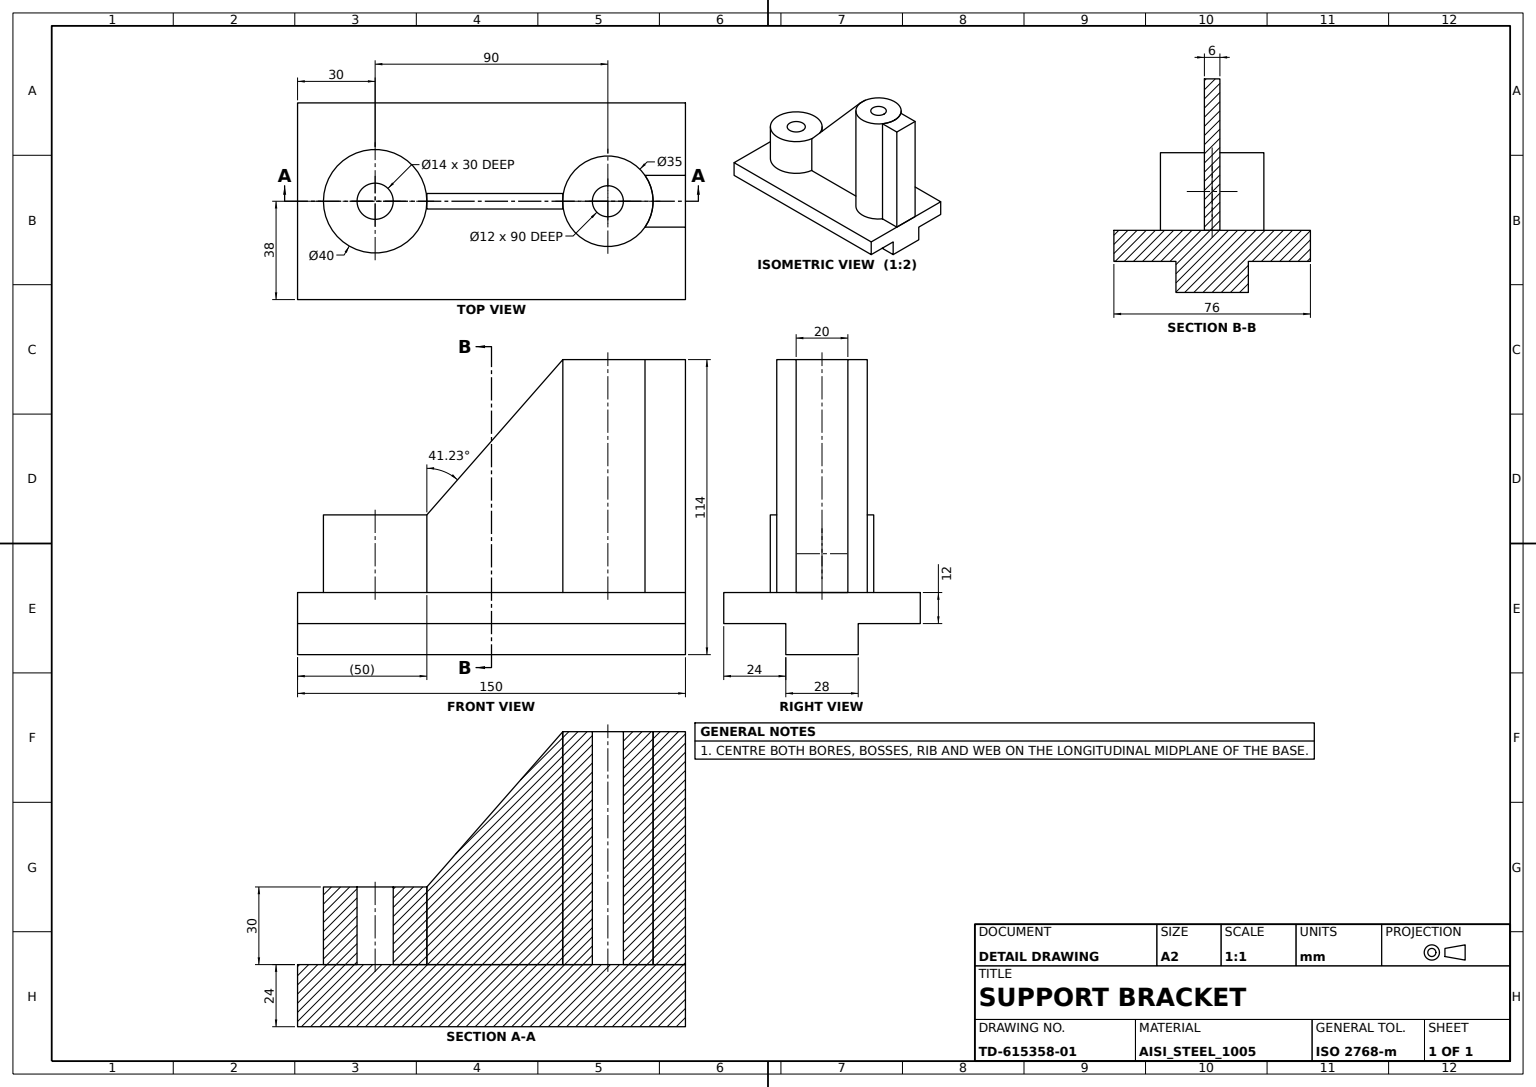
ISO-10303-21;
HEADER;
FILE_DESCRIPTION((''),'2;1');
FILE_NAME('','',(''),(''),'','','');
FILE_SCHEMA(('AUTOMOTIVE_DESIGN'));
ENDSEC;
DATA;
#1=APPLICATION_CONTEXT('');
#2=PRODUCT_CONTEXT('',#1,'mechanical');
#3=PRODUCT('','','',(#2));
#4=PRODUCT_DEFINITION_FORMATION('','',#3);
#5=PRODUCT_DEFINITION_CONTEXT('',#1,'design');
#6=PRODUCT_DEFINITION('','',#4,#5);
#7=PRODUCT_DEFINITION_SHAPE('','',#6);
#8=(LENGTH_UNIT()NAMED_UNIT(*)SI_UNIT(.MILLI.,.METRE.));
#9=(NAMED_UNIT(*)PLANE_ANGLE_UNIT()SI_UNIT($,.RADIAN.));
#10=(NAMED_UNIT(*)SI_UNIT($,.STERADIAN.)SOLID_ANGLE_UNIT());
#11=UNCERTAINTY_MEASURE_WITH_UNIT(LENGTH_MEASURE(0.005),#8,'distance_accuracy_value','');
#12=(GEOMETRIC_REPRESENTATION_CONTEXT(3)GLOBAL_UNCERTAINTY_ASSIGNED_CONTEXT((#11))GLOBAL_UNIT_ASSIGNED_CONTEXT((#8,#9,#10))REPRESENTATION_CONTEXT('',''));
#13=CARTESIAN_POINT('',(10.,-15.638593,114.));
#14=VERTEX_POINT('',#13);
#15=CARTESIAN_POINT('',(-10.,-15.638593,114.));
#16=VERTEX_POINT('',#15);
#17=CARTESIAN_POINT('',(0.,-30.,114.));
#18=DIRECTION('',(0.,0.,1.));
#19=DIRECTION('',(0.,1.,0.));
#20=AXIS2_PLACEMENT_3D('',#17,#18,#19);
#21=CIRCLE('',#20,17.5);
#22=EDGE_CURVE('',#14,#16,#21,.T.);
#23=ORIENTED_EDGE('',*,*,#22,.F.);
#24=CARTESIAN_POINT('',(10.,0.,114.));
#25=VERTEX_POINT('',#24);
#26=DIRECTION('',(0.,-1.,0.));
#27=VECTOR('',#26,1000.);
#28=LINE('',#24,#27);
#29=EDGE_CURVE('',#25,#14,#28,.T.);
#30=ORIENTED_EDGE('',*,*,#29,.F.);
#31=CARTESIAN_POINT('',(-10.,0.,114.));
#32=VERTEX_POINT('',#31);
#33=DIRECTION('',(1.,0.,0.));
#34=VECTOR('',#33,1000.);
#35=LINE('',#31,#34);
#36=EDGE_CURVE('',#32,#25,#35,.T.);
#37=ORIENTED_EDGE('',*,*,#36,.F.);
#38=VECTOR('',#19,1000.);
#39=LINE('',#15,#38);
#40=EDGE_CURVE('',#16,#32,#39,.T.);
#41=ORIENTED_EDGE('',*,*,#40,.F.);
#42=EDGE_LOOP('',(#23,#30,#37,#41));
#43=FACE_BOUND('',#42,.T.);
#44=AXIS2_PLACEMENT_3D('',#17,#18,#33);
#45=PLANE('',#44);
#46=ADVANCED_FACE('',(#43),#45,.T.);
#47=CARTESIAN_POINT('',(10.,-15.638593,24.));
#48=VERTEX_POINT('',#47);
#49=VECTOR('',#18,1000.);
#50=LINE('',#47,#49);
#51=EDGE_CURVE('',#48,#14,#50,.T.);
#52=ORIENTED_EDGE('',*,*,#51,.T.);
#53=ORIENTED_EDGE('',*,*,#22,.T.);
#54=CARTESIAN_POINT('',(-10.,-15.638593,24.));
#55=VERTEX_POINT('',#54);
#56=LINE('',#54,#49);
#57=EDGE_CURVE('',#55,#16,#56,.T.);
#58=ORIENTED_EDGE('',*,*,#57,.F.);
#59=CARTESIAN_POINT('',(0.,-30.,24.));
#60=AXIS2_PLACEMENT_3D('',#59,#18,#19);
#61=CIRCLE('',#60,17.5);
#62=EDGE_CURVE('',#48,#55,#61,.T.);
#63=ORIENTED_EDGE('',*,*,#62,.F.);
#64=EDGE_LOOP('',(#52,#53,#58,#63));
#65=FACE_BOUND('',#64,.T.);
#66=AXIS2_PLACEMENT_3D('',#59,#18,#33);
#67=CYLINDRICAL_SURFACE('',#66,17.5);
#68=ADVANCED_FACE('',(#65),#67,.F.);
#69=CARTESIAN_POINT('',(10.,0.,24.));
#70=VERTEX_POINT('',#69);
#71=LINE('',#69,#49);
#72=EDGE_CURVE('',#70,#25,#71,.T.);
#73=ORIENTED_EDGE('',*,*,#72,.T.);
#74=ORIENTED_EDGE('',*,*,#29,.T.);
#75=ORIENTED_EDGE('',*,*,#51,.F.);
#76=LINE('',#69,#27);
#77=EDGE_CURVE('',#70,#48,#76,.T.);
#78=ORIENTED_EDGE('',*,*,#77,.F.);
#79=EDGE_LOOP('',(#73,#74,#75,#78));
#80=FACE_BOUND('',#79,.T.);
#81=DIRECTION('',(-1.,0.,0.));
#82=AXIS2_PLACEMENT_3D('',#69,#81,#26);
#83=PLANE('',#82);
#84=ADVANCED_FACE('',(#80),#83,.F.);
#85=ORIENTED_EDGE('',*,*,#36,.T.);
#86=ORIENTED_EDGE('',*,*,#72,.F.);
#87=CARTESIAN_POINT('',(-10.,0.,24.));
#88=VERTEX_POINT('',#87);
#89=LINE('',#87,#34);
#90=EDGE_CURVE('',#88,#70,#89,.T.);
#91=ORIENTED_EDGE('',*,*,#90,.F.);
#92=LINE('',#87,#49);
#93=EDGE_CURVE('',#88,#32,#92,.T.);
#94=ORIENTED_EDGE('',*,*,#93,.T.);
#95=EDGE_LOOP('',(#85,#86,#91,#94));
#96=FACE_BOUND('',#95,.T.);
#97=DIRECTION('',(0.,0.,-1.));
#98=AXIS2_PLACEMENT_3D('',#87,#26,#97);
#99=PLANE('',#98);
#100=ADVANCED_FACE('',(#96),#99,.F.);
#101=LINE('',#54,#38);
#102=EDGE_CURVE('',#55,#88,#101,.T.);
#103=ORIENTED_EDGE('',*,*,#102,.F.);
#104=ORIENTED_EDGE('',*,*,#57,.T.);
#105=ORIENTED_EDGE('',*,*,#40,.T.);
#106=ORIENTED_EDGE('',*,*,#93,.F.);
#107=EDGE_LOOP('',(#103,#104,#105,#106));
#108=FACE_BOUND('',#107,.T.);
#109=AXIS2_PLACEMENT_3D('',#54,#33,#19);
#110=PLANE('',#109);
#111=ADVANCED_FACE('',(#108),#110,.F.);
#112=ORIENTED_EDGE('',*,*,#102,.T.);
#113=ORIENTED_EDGE('',*,*,#90,.T.);
#114=ORIENTED_EDGE('',*,*,#77,.T.);
#115=ORIENTED_EDGE('',*,*,#62,.T.);
#116=EDGE_LOOP('',(#112,#113,#114,#115));
#117=FACE_BOUND('',#116,.T.);
#118=PLANE('',#66);
#119=ADVANCED_FACE('',(#117),#118,.F.);
#120=CLOSED_SHELL('',(#46,#68,#84,#100,#111,#119));
#121=MANIFOLD_SOLID_BREP('',#120);
#122=CARTESIAN_POINT('',(-3.,-100.,54.));
#123=VERTEX_POINT('',#122);
#124=CARTESIAN_POINT('',(-3.,-47.413188,114.));
#125=VERTEX_POINT('',#124);
#126=DIRECTION('',(0.,0.659120652,0.75203721));
#127=VECTOR('',#126,1000.);
#128=LINE('',#122,#127);
#129=EDGE_CURVE('',#123,#125,#128,.T.);
#130=ORIENTED_EDGE('',*,*,#129,.F.);
#131=CARTESIAN_POINT('',(3.,-100.,54.));
#132=VERTEX_POINT('',#131);
#133=VECTOR('',#81,1000.);
#134=LINE('',#131,#133);
#135=EDGE_CURVE('',#132,#123,#134,.T.);
#136=ORIENTED_EDGE('',*,*,#135,.F.);
#137=CARTESIAN_POINT('',(3.,-47.413188,114.));
#138=VERTEX_POINT('',#137);
#139=LINE('',#131,#127);
#140=EDGE_CURVE('',#132,#138,#139,.T.);
#141=ORIENTED_EDGE('',*,*,#140,.T.);
#142=LINE('',#137,#133);
#143=EDGE_CURVE('',#138,#125,#142,.T.);
#144=ORIENTED_EDGE('',*,*,#143,.T.);
#145=EDGE_LOOP('',(#130,#136,#141,#144));
#146=FACE_BOUND('',#145,.T.);
#147=DIRECTION('',(0.,-0.75203721,0.659120652));
#148=DIRECTION('',(0.,-0.659120652,-0.75203721));
#149=AXIS2_PLACEMENT_3D('',#131,#147,#148);
#150=PLANE('',#149);
#151=ADVANCED_FACE('',(#146),#150,.T.);
#152=CARTESIAN_POINT('',(-3.,-100.,24.));
#153=VERTEX_POINT('',#152);
#154=LINE('',#152,#49);
#155=EDGE_CURVE('',#153,#123,#154,.T.);
#156=ORIENTED_EDGE('',*,*,#155,.T.);
#157=ORIENTED_EDGE('',*,*,#129,.T.);
#158=CARTESIAN_POINT('',(-3.,-47.413188,24.));
#159=VERTEX_POINT('',#158);
#160=VECTOR('',#97,1000.);
#161=LINE('',#124,#160);
#162=EDGE_CURVE('',#125,#159,#161,.T.);
#163=ORIENTED_EDGE('',*,*,#162,.T.);
#164=LINE('',#158,#27);
#165=EDGE_CURVE('',#159,#153,#164,.T.);
#166=ORIENTED_EDGE('',*,*,#165,.T.);
#167=EDGE_LOOP('',(#156,#157,#163,#166));
#168=FACE_BOUND('',#167,.T.);
#169=CARTESIAN_POINT('',(-3.,0.,0.));
#170=AXIS2_PLACEMENT_3D('',#169,#33,#97);
#171=PLANE('',#170);
#172=ADVANCED_FACE('',(#168),#171,.F.);
#173=ORIENTED_EDGE('',*,*,#140,.F.);
#174=CARTESIAN_POINT('',(3.,-100.,24.));
#175=VERTEX_POINT('',#174);
#176=LINE('',#174,#49);
#177=EDGE_CURVE('',#175,#132,#176,.T.);
#178=ORIENTED_EDGE('',*,*,#177,.F.);
#179=CARTESIAN_POINT('',(3.,-47.413188,24.));
#180=VERTEX_POINT('',#179);
#181=LINE('',#179,#27);
#182=EDGE_CURVE('',#180,#175,#181,.T.);
#183=ORIENTED_EDGE('',*,*,#182,.F.);
#184=LINE('',#137,#160);
#185=EDGE_CURVE('',#138,#180,#184,.T.);
#186=ORIENTED_EDGE('',*,*,#185,.F.);
#187=EDGE_LOOP('',(#173,#178,#183,#186));
#188=FACE_BOUND('',#187,.T.);
#189=CARTESIAN_POINT('',(3.,0.,0.));
#190=AXIS2_PLACEMENT_3D('',#189,#33,#97);
#191=PLANE('',#190);
#192=ADVANCED_FACE('',(#188),#191,.T.);
#193=LINE('',#179,#133);
#194=EDGE_CURVE('',#180,#159,#193,.T.);
#195=ORIENTED_EDGE('',*,*,#194,.T.);
#196=ORIENTED_EDGE('',*,*,#162,.F.);
#197=ORIENTED_EDGE('',*,*,#143,.F.);
#198=ORIENTED_EDGE('',*,*,#185,.T.);
#199=EDGE_LOOP('',(#195,#196,#197,#198));
#200=FACE_BOUND('',#199,.T.);
#201=AXIS2_PLACEMENT_3D('',#137,#19,#18);
#202=PLANE('',#201);
#203=ADVANCED_FACE('',(#200),#202,.T.);
#204=ORIENTED_EDGE('',*,*,#194,.F.);
#205=ORIENTED_EDGE('',*,*,#182,.T.);
#206=LINE('',#174,#133);
#207=EDGE_CURVE('',#175,#153,#206,.T.);
#208=ORIENTED_EDGE('',*,*,#207,.T.);
#209=ORIENTED_EDGE('',*,*,#165,.F.);
#210=EDGE_LOOP('',(#204,#205,#208,#209));
#211=FACE_BOUND('',#210,.T.);
#212=AXIS2_PLACEMENT_3D('',#179,#97,#81);
#213=PLANE('',#212);
#214=ADVANCED_FACE('',(#211),#213,.T.);
#215=ORIENTED_EDGE('',*,*,#177,.T.);
#216=ORIENTED_EDGE('',*,*,#135,.T.);
#217=ORIENTED_EDGE('',*,*,#155,.F.);
#218=ORIENTED_EDGE('',*,*,#207,.F.);
#219=EDGE_LOOP('',(#215,#216,#217,#218));
#220=FACE_BOUND('',#219,.T.);
#221=AXIS2_PLACEMENT_3D('',#174,#26,#97);
#222=PLANE('',#221);
#223=ADVANCED_FACE('',(#220),#222,.T.);
#224=CLOSED_SHELL('',(#151,#172,#192,#203,#214,#223));
#225=MANIFOLD_SOLID_BREP('',#224);
#226=CARTESIAN_POINT('',(0.,-113.,24.));
#227=VERTEX_POINT('',#226);
#228=CARTESIAN_POINT('',(0.,-120.,24.));
#229=AXIS2_PLACEMENT_3D('',#228,#18,#19);
#230=CIRCLE('',#229,7.);
#231=EDGE_CURVE('',#227,#227,#230,.T.);
#232=ORIENTED_EDGE('',*,*,#231,.T.);
#233=EDGE_LOOP('',(#232));
#234=FACE_BOUND('',#233,.T.);
#235=CARTESIAN_POINT('',(0.,-100.,24.));
#236=VERTEX_POINT('',#235);
#237=CIRCLE('',#229,20.);
#238=EDGE_CURVE('',#236,#236,#237,.T.);
#239=ORIENTED_EDGE('',*,*,#238,.F.);
#240=EDGE_LOOP('',(#239));
#241=FACE_BOUND('',#240,.T.);
#242=AXIS2_PLACEMENT_3D('',#228,#18,#33);
#243=PLANE('',#242);
#244=ADVANCED_FACE('',(#234,#241),#243,.F.);
#245=CARTESIAN_POINT('',(0.,-100.,54.));
#246=VERTEX_POINT('',#245);
#247=CARTESIAN_POINT('',(0.,-120.,54.));
#248=AXIS2_PLACEMENT_3D('',#247,#18,#19);
#249=CIRCLE('',#248,20.);
#250=EDGE_CURVE('',#246,#246,#249,.T.);
#251=ORIENTED_EDGE('',*,*,#250,.T.);
#252=EDGE_LOOP('',(#251));
#253=FACE_BOUND('',#252,.T.);
#254=CARTESIAN_POINT('',(0.,-113.,54.));
#255=VERTEX_POINT('',#254);
#256=CIRCLE('',#248,7.);
#257=EDGE_CURVE('',#255,#255,#256,.T.);
#258=ORIENTED_EDGE('',*,*,#257,.F.);
#259=EDGE_LOOP('',(#258));
#260=FACE_BOUND('',#259,.T.);
#261=AXIS2_PLACEMENT_3D('',#247,#18,#33);
#262=PLANE('',#261);
#263=ADVANCED_FACE('',(#253,#260),#262,.T.);
#264=ORIENTED_EDGE('',*,*,#257,.T.);
#265=EDGE_LOOP('',(#264));
#266=FACE_BOUND('',#265,.T.);
#267=ORIENTED_EDGE('',*,*,#231,.F.);
#268=EDGE_LOOP('',(#267));
#269=FACE_BOUND('',#268,.T.);
#270=AXIS2_PLACEMENT_3D('',#247,#97,#81);
#271=CYLINDRICAL_SURFACE('',#270,7.);
#272=ADVANCED_FACE('',(#266,#269),#271,.F.);
#273=ORIENTED_EDGE('',*,*,#250,.F.);
#274=EDGE_LOOP('',(#273));
#275=FACE_BOUND('',#274,.T.);
#276=ORIENTED_EDGE('',*,*,#238,.T.);
#277=EDGE_LOOP('',(#276));
#278=FACE_BOUND('',#277,.T.);
#279=CYLINDRICAL_SURFACE('',#270,20.);
#280=ADVANCED_FACE('',(#275,#278),#279,.T.);
#281=CLOSED_SHELL('',(#244,#263,#272,#280));
#282=MANIFOLD_SOLID_BREP('',#281);
#283=CARTESIAN_POINT('',(14.,-150.,12.));
#284=VERTEX_POINT('',#283);
#285=CARTESIAN_POINT('',(14.,0.,12.));
#286=VERTEX_POINT('',#285);
#287=LINE('',#283,#38);
#288=EDGE_CURVE('',#284,#286,#287,.T.);
#289=ORIENTED_EDGE('',*,*,#288,.T.);
#290=CARTESIAN_POINT('',(38.,0.,12.));
#291=VERTEX_POINT('',#290);
#292=LINE('',#290,#133);
#293=EDGE_CURVE('',#291,#286,#292,.T.);
#294=ORIENTED_EDGE('',*,*,#293,.F.);
#295=CARTESIAN_POINT('',(38.,-150.,12.));
#296=VERTEX_POINT('',#295);
#297=LINE('',#295,#38);
#298=EDGE_CURVE('',#296,#291,#297,.T.);
#299=ORIENTED_EDGE('',*,*,#298,.F.);
#300=LINE('',#295,#133);
#301=EDGE_CURVE('',#296,#284,#300,.T.);
#302=ORIENTED_EDGE('',*,*,#301,.T.);
#303=EDGE_LOOP('',(#289,#294,#299,#302));
#304=FACE_BOUND('',#303,.T.);
#305=AXIS2_PLACEMENT_3D('',#295,#97,#81);
#306=PLANE('',#305);
#307=ADVANCED_FACE('',(#304),#306,.T.);
#308=CARTESIAN_POINT('',(14.,0.,0.));
#309=VERTEX_POINT('',#308);
#310=CARTESIAN_POINT('',(-14.,0.,0.));
#311=VERTEX_POINT('',#310);
#312=LINE('',#308,#133);
#313=EDGE_CURVE('',#309,#311,#312,.T.);
#314=ORIENTED_EDGE('',*,*,#313,.F.);
#315=CARTESIAN_POINT('',(14.,-150.,0.));
#316=VERTEX_POINT('',#315);
#317=LINE('',#315,#38);
#318=EDGE_CURVE('',#316,#309,#317,.T.);
#319=ORIENTED_EDGE('',*,*,#318,.F.);
#320=CARTESIAN_POINT('',(-14.,-150.,0.));
#321=VERTEX_POINT('',#320);
#322=LINE('',#315,#133);
#323=EDGE_CURVE('',#316,#321,#322,.T.);
#324=ORIENTED_EDGE('',*,*,#323,.T.);
#325=LINE('',#320,#38);
#326=EDGE_CURVE('',#321,#311,#325,.T.);
#327=ORIENTED_EDGE('',*,*,#326,.T.);
#328=EDGE_LOOP('',(#314,#319,#324,#327));
#329=FACE_BOUND('',#328,.T.);
#330=AXIS2_PLACEMENT_3D('',#315,#97,#81);
#331=PLANE('',#330);
#332=ADVANCED_FACE('',(#329),#331,.T.);
#333=LINE('',#283,#160);
#334=EDGE_CURVE('',#284,#316,#333,.T.);
#335=ORIENTED_EDGE('',*,*,#334,.F.);
#336=ORIENTED_EDGE('',*,*,#301,.F.);
#337=CARTESIAN_POINT('',(38.,-150.,24.));
#338=VERTEX_POINT('',#337);
#339=LINE('',#337,#160);
#340=EDGE_CURVE('',#338,#296,#339,.T.);
#341=ORIENTED_EDGE('',*,*,#340,.F.);
#342=CARTESIAN_POINT('',(-38.,-150.,24.));
#343=VERTEX_POINT('',#342);
#344=LINE('',#342,#34);
#345=EDGE_CURVE('',#343,#338,#344,.T.);
#346=ORIENTED_EDGE('',*,*,#345,.F.);
#347=CARTESIAN_POINT('',(-38.,-150.,12.));
#348=VERTEX_POINT('',#347);
#349=LINE('',#347,#49);
#350=EDGE_CURVE('',#348,#343,#349,.T.);
#351=ORIENTED_EDGE('',*,*,#350,.F.);
#352=CARTESIAN_POINT('',(-14.,-150.,12.));
#353=VERTEX_POINT('',#352);
#354=LINE('',#352,#133);
#355=EDGE_CURVE('',#353,#348,#354,.T.);
#356=ORIENTED_EDGE('',*,*,#355,.F.);
#357=LINE('',#320,#49);
#358=EDGE_CURVE('',#321,#353,#357,.T.);
#359=ORIENTED_EDGE('',*,*,#358,.F.);
#360=ORIENTED_EDGE('',*,*,#323,.F.);
#361=EDGE_LOOP('',(#335,#336,#341,#346,#351,#356,#359,#360));
#362=FACE_BOUND('',#361,.T.);
#363=CARTESIAN_POINT('',(0.,-150.,0.));
#364=AXIS2_PLACEMENT_3D('',#363,#19,#18);
#365=PLANE('',#364);
#366=ADVANCED_FACE('',(#362),#365,.F.);
#367=CARTESIAN_POINT('',(38.,0.,24.));
#368=VERTEX_POINT('',#367);
#369=LINE('',#337,#38);
#370=EDGE_CURVE('',#338,#368,#369,.T.);
#371=ORIENTED_EDGE('',*,*,#370,.T.);
#372=CARTESIAN_POINT('',(-38.,0.,24.));
#373=VERTEX_POINT('',#372);
#374=LINE('',#372,#34);
#375=EDGE_CURVE('',#373,#368,#374,.T.);
#376=ORIENTED_EDGE('',*,*,#375,.F.);
#377=LINE('',#342,#38);
#378=EDGE_CURVE('',#343,#373,#377,.T.);
#379=ORIENTED_EDGE('',*,*,#378,.F.);
#380=ORIENTED_EDGE('',*,*,#345,.T.);
#381=EDGE_LOOP('',(#371,#376,#379,#380));
#382=FACE_BOUND('',#381,.T.);
#383=AXIS2_PLACEMENT_3D('',#342,#18,#33);
#384=PLANE('',#383);
#385=ADVANCED_FACE('',(#382),#384,.T.);
#386=CARTESIAN_POINT('',(-38.,0.,12.));
#387=VERTEX_POINT('',#386);
#388=LINE('',#347,#38);
#389=EDGE_CURVE('',#348,#387,#388,.T.);
#390=ORIENTED_EDGE('',*,*,#389,.F.);
#391=ORIENTED_EDGE('',*,*,#350,.T.);
#392=ORIENTED_EDGE('',*,*,#378,.T.);
#393=LINE('',#386,#49);
#394=EDGE_CURVE('',#387,#373,#393,.T.);
#395=ORIENTED_EDGE('',*,*,#394,.F.);
#396=EDGE_LOOP('',(#390,#391,#392,#395));
#397=FACE_BOUND('',#396,.T.);
#398=AXIS2_PLACEMENT_3D('',#347,#81,#18);
#399=PLANE('',#398);
#400=ADVANCED_FACE('',(#397),#399,.T.);
#401=ORIENTED_EDGE('',*,*,#370,.F.);
#402=ORIENTED_EDGE('',*,*,#340,.T.);
#403=ORIENTED_EDGE('',*,*,#298,.T.);
#404=LINE('',#367,#160);
#405=EDGE_CURVE('',#368,#291,#404,.T.);
#406=ORIENTED_EDGE('',*,*,#405,.F.);
#407=EDGE_LOOP('',(#401,#402,#403,#406));
#408=FACE_BOUND('',#407,.T.);
#409=AXIS2_PLACEMENT_3D('',#337,#33,#97);
#410=PLANE('',#409);
#411=ADVANCED_FACE('',(#408),#410,.T.);
#412=CARTESIAN_POINT('',(-14.,0.,12.));
#413=VERTEX_POINT('',#412);
#414=LINE('',#352,#38);
#415=EDGE_CURVE('',#353,#413,#414,.T.);
#416=ORIENTED_EDGE('',*,*,#415,.F.);
#417=ORIENTED_EDGE('',*,*,#355,.T.);
#418=ORIENTED_EDGE('',*,*,#389,.T.);
#419=LINE('',#412,#133);
#420=EDGE_CURVE('',#413,#387,#419,.T.);
#421=ORIENTED_EDGE('',*,*,#420,.F.);
#422=EDGE_LOOP('',(#416,#417,#418,#421));
#423=FACE_BOUND('',#422,.T.);
#424=AXIS2_PLACEMENT_3D('',#352,#97,#81);
#425=PLANE('',#424);
#426=ADVANCED_FACE('',(#423),#425,.T.);
#427=ORIENTED_EDGE('',*,*,#415,.T.);
#428=LINE('',#310,#49);
#429=EDGE_CURVE('',#311,#413,#428,.T.);
#430=ORIENTED_EDGE('',*,*,#429,.F.);
#431=ORIENTED_EDGE('',*,*,#326,.F.);
#432=ORIENTED_EDGE('',*,*,#358,.T.);
#433=EDGE_LOOP('',(#427,#430,#431,#432));
#434=FACE_BOUND('',#433,.T.);
#435=AXIS2_PLACEMENT_3D('',#320,#81,#18);
#436=PLANE('',#435);
#437=ADVANCED_FACE('',(#434),#436,.T.);
#438=LINE('',#285,#160);
#439=EDGE_CURVE('',#286,#309,#438,.T.);
#440=ORIENTED_EDGE('',*,*,#439,.T.);
#441=ORIENTED_EDGE('',*,*,#313,.T.);
#442=ORIENTED_EDGE('',*,*,#429,.T.);
#443=ORIENTED_EDGE('',*,*,#420,.T.);
#444=ORIENTED_EDGE('',*,*,#394,.T.);
#445=ORIENTED_EDGE('',*,*,#375,.T.);
#446=ORIENTED_EDGE('',*,*,#405,.T.);
#447=ORIENTED_EDGE('',*,*,#293,.T.);
#448=EDGE_LOOP('',(#440,#441,#442,#443,#444,#445,#446,#447));
#449=FACE_BOUND('',#448,.T.);
#450=CARTESIAN_POINT('',(0.,0.,0.));
#451=AXIS2_PLACEMENT_3D('',#450,#19,#18);
#452=PLANE('',#451);
#453=ADVANCED_FACE('',(#449),#452,.T.);
#454=ORIENTED_EDGE('',*,*,#318,.T.);
#455=ORIENTED_EDGE('',*,*,#439,.F.);
#456=ORIENTED_EDGE('',*,*,#288,.F.);
#457=ORIENTED_EDGE('',*,*,#334,.T.);
#458=EDGE_LOOP('',(#454,#455,#456,#457));
#459=FACE_BOUND('',#458,.T.);
#460=AXIS2_PLACEMENT_3D('',#283,#33,#97);
#461=PLANE('',#460);
#462=ADVANCED_FACE('',(#459),#461,.T.);
#463=CLOSED_SHELL('',(#307,#332,#366,#385,#400,#411,#426,#437,#453,#462));
#464=MANIFOLD_SOLID_BREP('',#463);
#465=CARTESIAN_POINT('',(0.,-12.5,24.));
#466=VERTEX_POINT('',#465);
#467=AXIS2_PLACEMENT_3D('',#59,#97,#19);
#468=CIRCLE('',#467,17.5);
#469=EDGE_CURVE('',#466,#466,#468,.T.);
#470=ORIENTED_EDGE('',*,*,#469,.F.);
#471=EDGE_LOOP('',(#470));
#472=FACE_BOUND('',#471,.T.);
#473=CARTESIAN_POINT('',(0.,-12.5,114.));
#474=VERTEX_POINT('',#473);
#475=AXIS2_PLACEMENT_3D('',#17,#97,#19);
#476=CIRCLE('',#475,17.5);
#477=EDGE_CURVE('',#474,#474,#476,.T.);
#478=ORIENTED_EDGE('',*,*,#477,.T.);
#479=EDGE_LOOP('',(#478));
#480=FACE_BOUND('',#479,.T.);
#481=AXIS2_PLACEMENT_3D('',#17,#97,#81);
#482=CYLINDRICAL_SURFACE('',#481,17.5);
#483=ADVANCED_FACE('',(#472,#480),#482,.T.);
#484=CARTESIAN_POINT('',(0.,-24.,24.));
#485=VERTEX_POINT('',#484);
#486=CIRCLE('',#467,6.);
#487=EDGE_CURVE('',#485,#485,#486,.T.);
#488=ORIENTED_EDGE('',*,*,#487,.T.);
#489=EDGE_LOOP('',(#488));
#490=FACE_BOUND('',#489,.T.);
#491=CARTESIAN_POINT('',(0.,-24.,114.));
#492=VERTEX_POINT('',#491);
#493=CIRCLE('',#475,6.);
#494=EDGE_CURVE('',#492,#492,#493,.T.);
#495=ORIENTED_EDGE('',*,*,#494,.F.);
#496=EDGE_LOOP('',(#495));
#497=FACE_BOUND('',#496,.T.);
#498=CYLINDRICAL_SURFACE('',#481,6.);
#499=ADVANCED_FACE('',(#490,#497),#498,.F.);
#500=ORIENTED_EDGE('',*,*,#477,.F.);
#501=EDGE_LOOP('',(#500));
#502=FACE_BOUND('',#501,.T.);
#503=ORIENTED_EDGE('',*,*,#494,.T.);
#504=EDGE_LOOP('',(#503));
#505=FACE_BOUND('',#504,.T.);
#506=PLANE('',#481);
#507=ADVANCED_FACE('',(#502,#505),#506,.F.);
#508=ORIENTED_EDGE('',*,*,#487,.F.);
#509=EDGE_LOOP('',(#508));
#510=FACE_BOUND('',#509,.T.);
#511=ORIENTED_EDGE('',*,*,#469,.T.);
#512=EDGE_LOOP('',(#511));
#513=FACE_BOUND('',#512,.T.);
#514=AXIS2_PLACEMENT_3D('',#59,#97,#81);
#515=PLANE('',#514);
#516=ADVANCED_FACE('',(#510,#513),#515,.T.);
#517=CLOSED_SHELL('',(#483,#499,#507,#516));
#518=MANIFOLD_SOLID_BREP('',#517);
#519=ADVANCED_BREP_SHAPE_REPRESENTATION('',(#121,#225,#282,#464,#518),#12);
#520=SHAPE_DEFINITION_REPRESENTATION(#7,#519);
ENDSEC;
END-ISO-10303-21;
